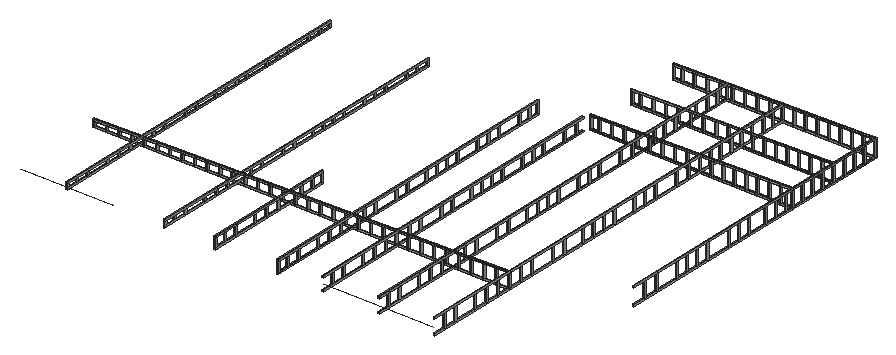
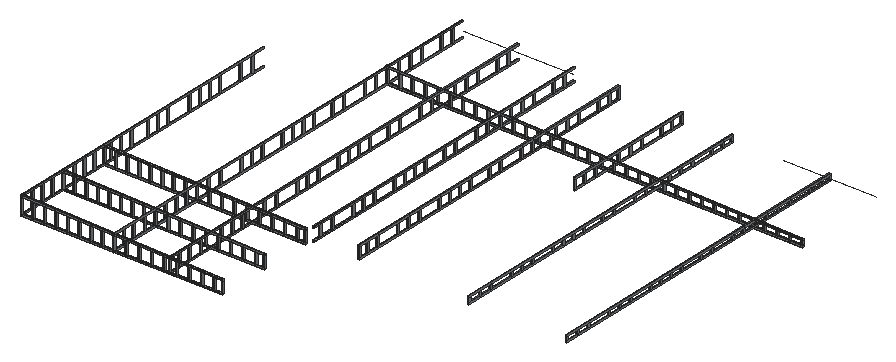
# SketchUp Ruby script. Lengths in millimetres.
U = 1.mm
M = Sketchup.active_model
def pt(a) = Geom::Point3d.new(a.map { |v| v * U })
def face(e, loops, mat)
  f = e.add_face(loops[0].map { |a| pt(a) })
  loops[1..].each { |l| e.add_face(l.map { |a| pt(a) }).erase! }
  f.material = f.back_material = mat if mat
  f
end
# faces: each face lists its corners as indices into pts; further lists are holes
def faces(e, pts, list, mat = nil) = list.each { |f| face(e, (f[0].is_a?(Array) ? f : [f]).map { |l| l.map { |i| pts[i] } }, mat) }
# xy, xz, yz: faces in a plane at the given z, y or x. An outline is a flat list of corners, or four numbers for a rectangle; further outlines are holes
def ring(l) = l.size == 4 ? [[l[0], l[1]], [l[2], l[1]], [l[2], l[3]], [l[0], l[3]]] : l.each_slice(2).to_a
def flat(e, list, mat, &to3) = list.each { |f| face(e, (f[0].is_a?(Array) ? f : [f]).map { |l| ring(l).map { |u, v| to3.(u, v) } }, mat) }
def xy(e, z, list, mat = nil) = flat(e, list, mat) { |x, y| [x, y, z] }
def xz(e, y, list, mat = nil) = flat(e, list, mat) { |x, z| [x, y, z] }
def yz(e, x, list, mat = nil) = flat(e, list, mat) { |y, z| [x, y, z] }
def lines(e, pts, list) = list.each { |a, b| e.add_line(pt(pts[a]), pt(pts[b])) }
# prism: a flat outline (further loops are holes) pulled along v
def prism(e, loops, v, mat = nil)
  f = face(e, loops, mat); d = Geom::Vector3d.new(v.map { |x| x * U })
  f.pushpull(f.normal.samedirection?(d) ? d.length : -d.length)
end
def box(e, o, s, mat = nil) = prism(e, [[o, [o[0] + s[0], o[1], o[2]], [o[0] + s[0], o[1] + s[1], o[2]], [o[0], o[1] + s[1], o[2]]]], [0, 0, s[2]], mat)
def at(x, y, z, deg = 0) = Geom::Transformation.translation(pt([x, y, z])) * Geom::Transformation.rotation(ORIGIN, Z_AXIS, deg.degrees)
def axes(o, x, y, z) = Geom::Transformation.new([*x, 0, *y, 0, *z, 0, *pt(o).to_a, 1])
def part(name) = M.definitions.add(name)
# library, detail: a bought-in or finely detailed component or shape, given as its bounding box
def library(name, o, s) = part(name).tap { |d| box(d.entities, o, s) }
def detail(e, o, s) = box(e.add_group.entities, o, s)
def put(e, d, t, mat = nil) = e.add_instance(d, t).tap { |i| i.material = mat if mat }
def group(e, t, mat = nil) = e.add_group.tap { |g| g.transformation = t; g.material = mat if mat }.entities
root = M.entities
M.materials.add("[Metal Rough]").color = [153, 157, 160]
c1 = part("Group\#8")
prism(c1.entities,[[[24013.3,85,80],[24013.3,85,831.9],[23933.3,85,830.1],[23933.3,85,80]]],[0,80,0],"[Metal Rough]")
prism(c1.entities,[[[20160.7,165,80],[20080.7,165,80],[20080.7,165,744.8],[20135.2,165,746],[20160.7,165,746.6]]],[0,-80,0],"[Metal Rough]")
prism(c1.entities,[[[20830,165,80],[20750,165,80],[20750,165,759.6],[20804.6,165,760.8],[20830,165,761.4]]],[0,-80,0],"[Metal Rough]")
prism(c1.entities,[[[18152.6,165,80],[18072.6,165,80],[18072.6,165,700.3],[18127.1,165,701.5],[18152.6,165,702.1]]],[0,-80,0],"[Metal Rough]")
prism(c1.entities,[[[21499.4,165,80],[21419.4,165,80],[21419.4,165,774.4],[21473.9,165,775.6],[21499.4,165,776.2]]],[0,-80,0],"[Metal Rough]")
prism(c1.entities,[[[19491.3,165,80],[19411.3,165,80],[19411.3,165,730],[19465.8,165,731.2],[19491.3,165,731.7]]],[0,-80,0],"[Metal Rough]")
prism(c1.entities,[[[16813.9,165,80],[16733.9,165,80],[16733.9,165,670.7],[16788.4,165,671.9],[16813.9,165,672.4]]],[0,-80,0],"[Metal Rough]")
prism(c1.entities,[[[16373.7,165,80],[16293.7,165,80],[16293.7,165,655.8],[16293.6,165,660.9],[16348.1,165,662.1],[16373.6,165,662.7],[16373.7,165,657.6]]],[0,-80,0],"[Metal Rough]")
prism(c1.entities,[[[17483.3,165,80],[17403.3,165,80],[17403.3,165,685.5],[17457.8,165,686.7],[17483.3,165,687.3]]],[0,-80,0],"[Metal Rough]")
prism(c1.entities,[[[18822,165,80],[18742,165,80],[18742,165,715.1],[18796.5,165,716.3],[18822,165,716.9]]],[0,-80,0],"[Metal Rough]")
prism(c1.entities,[[[27087.5,85,80],[27087.5,85,900],[27007.5,85,897.8],[27007.5,85,80]]],[0,80,0],"[Metal Rough]")
prism(c1.entities,[[[26472.7,165,80],[26392.7,165,80],[26392.7,165,884.6],[26472.7,165,886.4]]],[0,-80,0],"[Metal Rough]")
prism(c1.entities,[[[25857.8,165,80],[25777.8,165,80],[25777.8,165,871],[25857.8,165,872.8]]],[0,-80,0],"[Metal Rough]")
prism(c1.entities,[[[22168.7,165,80],[22088.7,165,80],[22088.8,165,789.3],[22168.8,165,791]]],[0,-80,0],"[Metal Rough]")
prism(c1.entities,[[[25243,165,80],[25163,165,80],[25163,165,857.4],[25243,165,859.1]]],[0,-80,0],"[Metal Rough]")
prism(c1.entities,[[[24628.1,165,80],[24548.1,165,80],[24548.1,165,843.7],[24628.1,165,845.5]]],[0,-80,0],"[Metal Rough]")
prism(c1.entities,[[[22783.6,85,80],[22783.6,85,804.7],[22703.6,85,802.9],[22703.6,85,80]]],[0,80,0],"[Metal Rough]")
prism(c1.entities,[[[23398.4,165,80],[23318.4,165,80],[23318.4,165,816.5],[23398.4,165,818.3]]],[0,-80,0],"[Metal Rough]")
p = [[21499.4,85,776.2],[21553.9,85,777.4]]
lines(c1.entities,p,[[0,1]])
g1 = group(c1.entities,at(0,85,0),"[Metal Rough]")
g2 = group(g1,at(0,0,300))
prism(g2,[[[27087.5,80,600],[16293.7,80,360.9],[16293.7,80,440.9],[27087.5,80,680]]],[0,-80,0])
g3 = group(g1,at(27087.5,0,0),"[Metal Rough]")
xy(g3,0,[[-10793.8,0,0,80]])
xy(g3,4,[[-10793.8,4,0,76]])
xy(g3,76,[[-10793.8,4,0,76]])
xy(g3,80,[[-10793.8,0,0,80]])
xz(g3,0,[[-10793.8,0,0,80]])
xz(g3,4,[[-10793.8,4,0,76]])
xz(g3,80,[[-10793.8,0,0,80]])
yz(g3,-10793.8,[[0,0,0,80,80,80,80,76,4,76,4,4,80,4,80,0],[4,4,80,76]])
yz(g3,0,[[[0,0,80,80],[4,4,76,76]]])
c2 = part("Group\#51")
box(c2.entities,[0,0,0],[80,17322.9,80])
c3 = part("Group\#46")
box(c3.entities,[0,0,0],[80,17322.9,80])
c4 = part("Group\#57")
box(c4.entities,[0,0,0],[80,80,820])
c5 = part("Group\#52")
box(c5.entities,[0,0,0],[80,23204,80])
c6 = part("Group\#7")
prism(c6.entities,[[[0,0,4955],[0,80,4955],[80,80,4955],[80,0,4955]],[[76,76,4955],[4,76,4955],[4,4,4955],[76,4,4955]]],[0,0,22132.5])
c7 = part("Group\#29")
box(c7.entities,[0,0,0],[80,16119.2,80])
c8 = part("Group\#49")
box(c8.entities,[0,0,0],[80,17546,80])
c9 = part("Group\#48")
box(c9.entities,[0,0,0],[80,17546,80])
p = [[17973.9,2438,3368.8],[23848.8,2438,3368.8],[1836.3,2438,3190.9],[6789.8,2438,3190.9]]
lines(root,p,[[0,1],[2,3]])
put(root,c1,at(1752.5,22725.5,3000))
g4 = group(root,at(15500.9,2438,3000))
put(g4,c2,at(0,0,0),"[Metal Rough]")
put(g4,c3,at(0,0,606.2),"[Metal Rough]")
put(g4,c4,axes([0,1326.8,80],[1,0,0],[0,1,0],[0,0,0.64174]),"[Metal Rough]")
put(g4,c4,axes([0,619.8,80],[1,0,0],[0,1,0],[0,0,0.64174]),"[Metal Rough]")
put(g4,c4,axes([0,2630.8,80],[1,0,0],[0,1,0],[0,0,0.64174]),"[Metal Rough]")
put(g4,c4,axes([0,3409.8,80],[1,0,0],[0,1,0],[0,0,0.64174]),"[Metal Rough]")
put(g4,c4,axes([0,4163.8,80],[1,0,0],[0,1,0],[0,0,0.64174]),"[Metal Rough]")
put(g4,c4,axes([0,5701.8,80],[1,0,0],[0,1,0],[0,0,0.64174]),"[Metal Rough]")
put(g4,c4,axes([0,6439.8,80],[1,0,0],[0,1,0],[0,0,0.64174]),"[Metal Rough]")
put(g4,c4,axes([0,8583.8,80],[1,0,0],[0,1,0],[0,0,0.64174]),"[Metal Rough]")
put(g4,c4,axes([0,7834.8,80],[1,0,0],[0,1,0],[0,0,0.64174]),"[Metal Rough]")
put(g4,c4,axes([0,9830.8,80],[1,0,0],[0,1,0],[0,0,0.64174]),"[Metal Rough]")
put(g4,c4,axes([0,10547.8,80],[1,0,0],[0,1,0],[0,0,0.64174]),"[Metal Rough]")
put(g4,c4,axes([0,11219.8,80],[1,0,0],[0,1,0],[0,0,0.64174]),"[Metal Rough]")
put(g4,c4,axes([0,11903.8,80],[1,0,0],[0,1,0],[0,0,0.64174]),"[Metal Rough]")
put(g4,c4,axes([0,13240.8,80],[1,0,0],[0,1,0],[0,0,0.64174]),"[Metal Rough]")
put(g4,c4,axes([0,13957.8,80],[1,0,0],[0,1,0],[0,0,0.64174]),"[Metal Rough]")
put(g4,c4,axes([0,14664.8,80],[1,0,0],[0,1,0],[0,0,0.64174]),"[Metal Rough]")
put(g4,c4,axes([0,16044.8,80],[1,0,0],[0,1,0],[0,0,0.64174]),"[Metal Rough]")
put(g4,c4,axes([0,16680.8,80],[1,0,0],[0,1,0],[0,0,0.64174]),"[Metal Rough]")
put(g4,c4,axes([0,0,80],[1,0,0],[0,1,0],[0,0,0.64174]),"[Metal Rough]")
put(g4,c4,axes([0,17242.9,80],[1,0,0],[0,1,0],[0,0,0.64174]),"[Metal Rough]")
put(root,c1,at(1756.3,19974,3000))
put(root,c1,at(1756.3,25477,3000))
g5 = group(root,at(17893.9,2438,3000))
put(g5,c2,at(0,0,0),"[Metal Rough]")
put(g5,c3,at(0,0,659.2),"[Metal Rough]")
put(g5,c4,axes([0,1326.8,80],[1,0,0],[0,1,0],[0,0,0.70638]),"[Metal Rough]")
put(g5,c4,axes([0,619.8,80],[1,0,0],[0,1,0],[0,0,0.70638]),"[Metal Rough]")
put(g5,c4,axes([0,2630.8,80],[1,0,0],[0,1,0],[0,0,0.70638]),"[Metal Rough]")
put(g5,c4,axes([0,3409.8,80],[1,0,0],[0,1,0],[0,0,0.70638]),"[Metal Rough]")
put(g5,c4,axes([0,4163.8,80],[1,0,0],[0,1,0],[0,0,0.70638]),"[Metal Rough]")
put(g5,c4,axes([0,5701.8,80],[1,0,0],[0,1,0],[0,0,0.70638]),"[Metal Rough]")
put(g5,c4,axes([0,6439.8,80],[1,0,0],[0,1,0],[0,0,0.70638]),"[Metal Rough]")
put(g5,c4,axes([0,8583.8,80],[1,0,0],[0,1,0],[0,0,0.70638]),"[Metal Rough]")
put(g5,c4,axes([0,7834.8,80],[1,0,0],[0,1,0],[0,0,0.70638]),"[Metal Rough]")
put(g5,c4,axes([0,9830.8,80],[1,0,0],[0,1,0],[0,0,0.70638]),"[Metal Rough]")
put(g5,c4,axes([0,10547.8,80],[1,0,0],[0,1,0],[0,0,0.70638]),"[Metal Rough]")
put(g5,c4,axes([0,11219.8,80],[1,0,0],[0,1,0],[0,0,0.70638]),"[Metal Rough]")
put(g5,c4,axes([0,11903.8,80],[1,0,0],[0,1,0],[0,0,0.70638]),"[Metal Rough]")
put(g5,c4,axes([0,13240.8,80],[1,0,0],[0,1,0],[0,0,0.70638]),"[Metal Rough]")
put(g5,c4,axes([0,13957.8,80],[1,0,0],[0,1,0],[0,0,0.70638]),"[Metal Rough]")
put(g5,c4,axes([0,14664.8,80],[1,0,0],[0,1,0],[0,0,0.70638]),"[Metal Rough]")
put(g5,c4,axes([0,16044.8,80],[1,0,0],[0,1,0],[0,0,0.70638]),"[Metal Rough]")
put(g5,c4,axes([0,16860.8,80],[1,0,0],[0,1,0],[0,0,0.70638]),"[Metal Rough]")
g6 = group(root,at(20871.3,2438,3000))
put(g6,c5,at(0,0,0),"[Metal Rough]")
put(g6,c5,at(0,0,725.2),"[Metal Rough]")
put(g6,c4,axes([0,1326.8,80],[1,0,0],[0,1,0],[0,0,0.78681]),"[Metal Rough]")
put(g6,c4,axes([0,619.8,80],[1,0,0],[0,1,0],[0,0,0.78681]),"[Metal Rough]")
put(g6,c4,axes([0,2630.8,80],[1,0,0],[0,1,0],[0,0,0.78681]),"[Metal Rough]")
put(g6,c4,axes([0,3409.8,80],[1,0,0],[0,1,0],[0,0,0.78681]),"[Metal Rough]")
put(g6,c4,axes([0,4163.8,80],[1,0,0],[0,1,0],[0,0,0.78681]),"[Metal Rough]")
put(g6,c4,axes([0,5701.8,80],[1,0,0],[0,1,0],[0,0,0.78681]),"[Metal Rough]")
put(g6,c4,axes([0,6439.8,80],[1,0,0],[0,1,0],[0,0,0.78681]),"[Metal Rough]")
put(g6,c4,axes([0,8583.8,80],[1,0,0],[0,1,0],[0,0,0.78681]),"[Metal Rough]")
put(g6,c4,axes([0,7834.8,80],[1,0,0],[0,1,0],[0,0,0.78681]),"[Metal Rough]")
put(g6,c4,axes([0,9830.8,80],[1,0,0],[0,1,0],[0,0,0.78681]),"[Metal Rough]")
put(g6,c4,axes([0,10547.8,80],[1,0,0],[0,1,0],[0,0,0.78681]),"[Metal Rough]")
put(g6,c4,axes([0,11219.8,80],[1,0,0],[0,1,0],[0,0,0.78681]),"[Metal Rough]")
put(g6,c4,axes([0,11903.8,80],[1,0,0],[0,1,0],[0,0,0.78681]),"[Metal Rough]")
put(g6,c4,axes([0,13240.8,80],[1,0,0],[0,1,0],[0,0,0.78681]),"[Metal Rough]")
put(g6,c4,axes([0,13957.8,80],[1,0,0],[0,1,0],[0,0,0.78681]),"[Metal Rough]")
put(g6,c4,axes([0,14664.8,80],[1,0,0],[0,1,0],[0,0,0.78681]),"[Metal Rough]")
put(g6,c4,axes([0,16044.8,80],[1,0,0],[0,1,0],[0,0,0.78681]),"[Metal Rough]")
put(g6,c4,axes([0,16860.8,80],[1,0,0],[0,1,0],[0,0,0.78681]),"[Metal Rough]")
put(g6,c4,axes([0,18313.8,80],[1,0,0],[0,1,0],[0,0,0.78681]),"[Metal Rough]")
put(g6,c4,axes([0,19693.8,80],[1,0,0],[0,1,0],[0,0,0.78681]),"[Metal Rough]")
put(g6,c4,axes([0,18980.8,80],[1,0,0],[0,1,0],[0,0,0.78681]),"[Metal Rough]")
put(g6,c4,axes([0,21064.8,80],[1,0,0],[0,1,0],[0,0,0.78681]),"[Metal Rough]")
put(g6,c4,axes([0,21831.8,80],[1,0,0],[0,1,0],[0,0,0.78681]),"[Metal Rough]")
put(g6,c4,axes([0,22478.8,80],[1,0,0],[0,1,0],[0,0,0.78681]),"[Metal Rough]")
put(g6,c4,axes([0,23124,80],[1,0,0],[0,1,0],[0,0,0.78681]),"[Metal Rough]")
g7 = group(root,at(23848.8,2438,3000))
put(g7,c5,at(0,0,0),"[Metal Rough]")
put(g7,c5,at(0,0,789.4),"[Metal Rough]")
put(g7,c4,axes([0,1326.8,80],[1,0,0],[0,1,0],[0,0,0.86507]),"[Metal Rough]")
put(g7,c4,axes([0,619.8,80],[1,0,0],[0,1,0],[0,0,0.86507]),"[Metal Rough]")
put(g7,c4,axes([0,2630.8,80],[1,0,0],[0,1,0],[0,0,0.86507]),"[Metal Rough]")
put(g7,c4,axes([0,3409.8,80],[1,0,0],[0,1,0],[0,0,0.86507]),"[Metal Rough]")
put(g7,c4,axes([0,4163.8,80],[1,0,0],[0,1,0],[0,0,0.86507]),"[Metal Rough]")
put(g7,c4,axes([0,5701.8,80],[1,0,0],[0,1,0],[0,0,0.86507]),"[Metal Rough]")
put(g7,c4,axes([0,6439.8,80],[1,0,0],[0,1,0],[0,0,0.86507]),"[Metal Rough]")
put(g7,c4,axes([0,8583.8,80],[1,0,0],[0,1,0],[0,0,0.86507]),"[Metal Rough]")
put(g7,c4,axes([0,7834.8,80],[1,0,0],[0,1,0],[0,0,0.86507]),"[Metal Rough]")
put(g7,c4,axes([0,9830.8,80],[1,0,0],[0,1,0],[0,0,0.86507]),"[Metal Rough]")
put(g7,c4,axes([0,10547.8,80],[1,0,0],[0,1,0],[0,0,0.86507]),"[Metal Rough]")
put(g7,c4,axes([0,11219.8,80],[1,0,0],[0,1,0],[0,0,0.86507]),"[Metal Rough]")
put(g7,c4,axes([0,11903.8,80],[1,0,0],[0,1,0],[0,0,0.86507]),"[Metal Rough]")
put(g7,c4,axes([0,13240.8,80],[1,0,0],[0,1,0],[0,0,0.86507]),"[Metal Rough]")
put(g7,c4,axes([0,13957.8,80],[1,0,0],[0,1,0],[0,0,0.86507]),"[Metal Rough]")
put(g7,c4,axes([0,14664.8,80],[1,0,0],[0,1,0],[0,0,0.86507]),"[Metal Rough]")
put(g7,c4,axes([0,16044.8,80],[1,0,0],[0,1,0],[0,0,0.86507]),"[Metal Rough]")
put(g7,c4,axes([0,16860.8,80],[1,0,0],[0,1,0],[0,0,0.86507]),"[Metal Rough]")
put(g7,c4,axes([0,18313.8,80],[1,0,0],[0,1,0],[0,0,0.86507]),"[Metal Rough]")
put(g7,c4,axes([0,19693.8,80],[1,0,0],[0,1,0],[0,0,0.86507]),"[Metal Rough]")
put(g7,c4,axes([0,18980.8,80],[1,0,0],[0,1,0],[0,0,0.86507]),"[Metal Rough]")
put(g7,c4,axes([0,21064.8,80],[1,0,0],[0,1,0],[0,0,0.86507]),"[Metal Rough]")
put(g7,c4,axes([0,21831.8,80],[1,0,0],[0,1,0],[0,0,0.86507]),"[Metal Rough]")
put(g7,c4,axes([0,22478.8,80],[1,0,0],[0,1,0],[0,0,0.86507]),"[Metal Rough]")
g8 = group(root,at(12150,2438,3000))
g9 = group(g8,at(0,0,0),"[Metal Rough]")
box(g9,[0,0,0],[80,7145.8,80])
g10 = group(g8,at(0,0,532),"[Metal Rough]")
box(g10,[0,0,0],[80,7145.8,80])
put(g8,c4,axes([0,1326.8,80],[1,0,0],[0,1,0],[0,0,0.55122]),"[Metal Rough]")
put(g8,c4,axes([0,619.8,80],[1,0,0],[0,1,0],[0,0,0.55122]),"[Metal Rough]")
put(g8,c4,axes([0,2630.8,80],[1,0,0],[0,1,0],[0,0,0.55122]),"[Metal Rough]")
put(g8,c4,axes([0,3409.8,80],[1,0,0],[0,1,0],[0,0,0.55122]),"[Metal Rough]")
put(g8,c4,axes([0,4163.8,80],[1,0,0],[0,1,0],[0,0,0.55122]),"[Metal Rough]")
put(g8,c4,axes([0,5701.8,80],[1,0,0],[0,1,0],[0,0,0.55122]),"[Metal Rough]")
put(g8,c4,axes([0,6439.8,80],[1,0,0],[0,1,0],[0,0,0.55122]),"[Metal Rough]")
put(g8,c4,axes([0,7084.8,80],[1,0,0],[0,1,0],[0,0,0.55122]),"[Metal Rough]")
put(g8,c4,axes([0,0,80],[1,0,0],[0,1,0],[0,0,0.55122]),"[Metal Rough]")
g11 = group(root,at(1756.3,7283,3000))
prism(g11,[[[6104.2,85,80],[6104.2,85,435.2],[6078.7,85,434.6],[6024.2,85,433.4],[6024.2,85,80]]],[0,80,0],"[Metal Rough]")
prism(g11,[[[7442.9,85,80],[7442.9,85,464.9],[7417.4,85,464.3],[7362.9,85,463.1],[7362.9,85,80]]],[0,80,0],"[Metal Rough]")
prism(g11,[[[6773.6,85,80],[6773.6,85,450],[6748.1,85,449.5],[6693.6,85,448.3],[6693.6,85,80]]],[0,80,0],"[Metal Rough]")
prism(g11,[[[8112.3,85,80],[8112.3,85,479.7],[8086.8,85,479.1],[8032.3,85,477.9],[8032.3,85,80]]],[0,80,0],"[Metal Rough]")
prism(g11,[[[5434.8,85,80],[5434.8,85,420.4],[5409.4,85,419.8],[5354.8,85,418.6],[5354.8,85,80]]],[0,80,0],"[Metal Rough]")
prism(g11,[[[4096.1,85,80],[4096.1,85,390.7],[4070.6,85,390.2],[4016.1,85,388.9],[4016.1,85,80]]],[0,80,0],"[Metal Rough]")
prism(g11,[[[1418.7,165,80],[1338.7,165,80],[1338.7,165,329.6],[1393.2,165,330.9],[1418.7,165,331.4]]],[0,-80,0],"[Metal Rough]")
prism(g11,[[[3426.8,165,80],[3346.8,165,80],[3346.8,165,374.1],[3401.3,165,375.3],[3426.8,165,375.9]]],[0,-80,0],"[Metal Rough]")
prism(g11,[[[2757.4,165,80],[2677.4,165,80],[2677.4,165,359.3],[2731.9,165,360.5],[2757.4,165,361.1]]],[0,-80,0],"[Metal Rough]")
prism(g11,[[[2088.1,165,80],[2008.1,165,80],[2008.1,165,344.5],[2062.6,165,345.7],[2088.1,165,346.2]]],[0,-80,0],"[Metal Rough]")
prism(g11,[[[4765.5,85,80],[4765.5,85,405.5],[4740,85,405],[4685.5,85,403.8],[4685.5,85,80]]],[0,80,0],"[Metal Rough]")
prism(g11,[[[80,85,80],[80,85,301.8],[0,85,300],[0,85,80]]],[0,80,0],"[Metal Rough]")
prism(g11,[[[749.4,85,80],[749.4,85,316.6],[669.4,85,314.8],[669.4,85,80]]],[0,80,0],"[Metal Rough]")
prism(g11,[[[12128.4,85,80],[12128.4,85,568.6],[12102.9,85,568.1],[12048.4,85,566.9],[12048.4,85,80]]],[0,80,0],"[Metal Rough]")
prism(g11,[[[10120.3,165,80],[10040.3,165,80],[10040.3,165,522.4],[10094.9,165,523.6],[10120.3,165,524.2]]],[0,-80,0],"[Metal Rough]")
prism(g11,[[[12797.8,85,80],[12797.8,85,583.5],[12772.3,85,582.9],[12717.8,85,581.7],[12717.8,85,80]]],[0,80,0],"[Metal Rough]")
prism(g11,[[[20160.7,165,80],[20080.7,165,80],[20080.7,165,744.8],[20135.2,165,746],[20160.7,165,746.6]]],[0,-80,0],"[Metal Rough]")
prism(g11,[[[20830,165,80],[20750,165,80],[20750,165,759.6],[20804.6,165,760.8],[20830,165,761.4]]],[0,-80,0],"[Metal Rough]")
prism(g11,[[[18152.6,165,80],[18072.6,165,80],[18072.6,165,700.3],[18127.1,165,701.5],[18152.6,165,702.1]]],[0,-80,0],"[Metal Rough]")
prism(g11,[[[21499.4,165,80],[21419.4,165,80],[21419.4,165,774.4],[21473.9,165,775.6],[21499.4,165,776.2]]],[0,-80,0],"[Metal Rough]")
prism(g11,[[[15475.2,165,80],[15395.2,165,80],[15395.2,165,641],[15449.7,165,642.2],[15475.2,165,642.8]]],[0,-80,0],"[Metal Rough]")
prism(g11,[[[19491.3,165,80],[19411.3,165,80],[19411.3,165,730],[19465.8,165,731.2],[19491.3,165,731.7]]],[0,-80,0],"[Metal Rough]")
prism(g11,[[[16813.9,165,80],[16733.9,165,80],[16733.9,165,670.7],[16788.4,165,671.9],[16813.9,165,672.4]]],[0,-80,0],"[Metal Rough]")
prism(g11,[[[16144.5,165,80],[16064.5,165,80],[16064.5,165,655.8],[16119.1,165,657],[16144.5,165,657.6]]],[0,-80,0],"[Metal Rough]")
prism(g11,[[[17483.3,165,80],[17403.3,165,80],[17403.3,165,685.5],[17457.8,165,686.7],[17483.3,165,687.3]]],[0,-80,0],"[Metal Rough]")
prism(g11,[[[14805.8,165,80],[14725.8,165,80],[14725.8,165,626.2],[14780.3,165,627.4],[14805.8,165,627.9]]],[0,-80,0],"[Metal Rough]")
prism(g11,[[[18822,165,80],[18742,165,80],[18742,165,715.1],[18796.5,165,716.3],[18822,165,716.9]]],[0,-80,0],"[Metal Rough]")
prism(g11,[[[10789.7,165,80],[10709.7,165,80],[10709.7,165,537.2],[10764.2,165,538.4],[10789.7,165,539]]],[0,-80,0],"[Metal Rough]")
prism(g11,[[[8781.6,165,80],[8701.6,165,80],[8701.6,165,492.7],[8756.1,165,493.9],[8781.6,165,494.5]]],[0,-80,0],"[Metal Rough]")
prism(g11,[[[9451,165,80],[9371,165,80],[9371,165,507.6],[9425.5,165,508.8],[9451,165,509.3]]],[0,-80,0],"[Metal Rough]")
prism(g11,[[[13467.1,165,80],[13387.1,165,80],[13387.1,165,596.5],[13441.6,165,597.7],[13467.1,165,598.3]]],[0,-80,0],"[Metal Rough]")
prism(g11,[[[14136.5,165,80],[14056.5,165,80],[14056.5,165,611.3],[14111,165,612.6],[14136.5,165,613.1]]],[0,-80,0],"[Metal Rough]")
prism(g11,[[[11459.1,165,80],[11379.1,165,80],[11379.1,165,552],[11433.6,165,553.2],[11459.1,165,553.8]]],[0,-80,0],"[Metal Rough]")
prism(g11,[[[22172.5,165,80],[22092.5,165,80],[22092.5,165,788.5],[22172.5,165,790.2]]],[0,-80,0],"[Metal Rough]")
p = [[21499.4,85,776.2],[21553.9,85,777.4]]
lines(g11,p,[[0,1]])
g12 = group(g11,at(0,85,0),"[Metal Rough]")
g13 = group(g12,at(0,0,300))
prism(g13,[[[0,80,80],[22132.5,80,570.3],[22172.5,80,570.3],[22172.5,80,490.2],[22132.5,80,490.2],[0,80,0]]],[0,-80,0])
put(g12,c6,axes([27087.5,0,0],[0,0,1],[0,1,0],[-1,0,0]),"[Metal Rough]")
g14 = group(root,at(28763.8,9522.8,3000))
g15 = group(g14,at(0,11217.2,80))
put(g15,c4,at(0,1336,0),"[Metal Rough]")
put(g15,c4,at(0,2775,0),"[Metal Rough]")
put(g15,c4,at(0,4111,0),"[Metal Rough]")
put(g15,c4,at(0,3443,0),"[Metal Rough]")
put(g15,c4,at(0,668,0),"[Metal Rough]")
put(g15,c4,at(0,0,0),"[Metal Rough]")
put(g15,c4,at(0,-1117,0),"[Metal Rough]")
put(g15,c4,at(0,-1785,0),"[Metal Rough]")
put(g15,c4,at(0,-2453,0),"[Metal Rough]")
put(g15,c4,at(0,-4232,0),"[Metal Rough]")
put(g15,c4,at(0,-3564,0),"[Metal Rough]")
put(g15,c4,at(0,-4900,0),"[Metal Rough]")
put(g15,c4,at(0,-7693,0),"[Metal Rough]")
put(g15,c4,at(0,-7025,0),"[Metal Rough]")
put(g15,c4,at(0,-6357,0),"[Metal Rough]")
put(g15,c4,at(0,-8364,0),"[Metal Rough]")
put(g15,c4,at(0,-9727,0),"[Metal Rough]")
put(g15,c4,at(0,-10515,0),"[Metal Rough]")
put(g14,c7,at(0,0,900),"[Metal Rough]")
put(g14,c7,at(0,0,0),"[Metal Rough]")
g16 = group(root,at(4273,2438,3080))
put(g16,c8,at(0,0,0),"[Metal Rough]")
put(g16,c9,at(0,0,277.5),"[Metal Rough]")
put(g16,c4,axes([0,1326.8,80],[1,0,0],[0,1,0],[0,0,0.24089]),"[Metal Rough]")
put(g16,c4,axes([0,619.8,80],[1,0,0],[0,1,0],[0,0,0.24089]),"[Metal Rough]")
put(g16,c4,axes([0,2630.8,80],[1,0,0],[0,1,0],[0,0,0.24089]),"[Metal Rough]")
put(g16,c4,axes([0,3409.8,80],[1,0,0],[0,1,0],[0,0,0.24089]),"[Metal Rough]")
put(g16,c4,axes([0,4163.8,80],[1,0,0],[0,1,0],[0,0,0.24089]),"[Metal Rough]")
put(g16,c4,axes([0,5701.8,80],[1,0,0],[0,1,0],[0,0,0.24089]),"[Metal Rough]")
put(g16,c4,axes([0,6439.8,80],[1,0,0],[0,1,0],[0,0,0.24089]),"[Metal Rough]")
put(g16,c4,axes([0,8583.8,80],[1,0,0],[0,1,0],[0,0,0.24089]),"[Metal Rough]")
put(g16,c4,axes([0,7834.8,80],[1,0,0],[0,1,0],[0,0,0.24089]),"[Metal Rough]")
put(g16,c4,axes([0,9830.8,80],[1,0,0],[0,1,0],[0,0,0.24089]),"[Metal Rough]")
put(g16,c4,axes([0,10547.8,80],[1,0,0],[0,1,0],[0,0,0.24089]),"[Metal Rough]")
put(g16,c4,axes([0,11219.8,80],[1,0,0],[0,1,0],[0,0,0.24089]),"[Metal Rough]")
put(g16,c4,axes([0,11903.8,80],[1,0,0],[0,1,0],[0,0,0.24089]),"[Metal Rough]")
put(g16,c4,axes([0,13240.8,80],[1,0,0],[0,1,0],[0,0,0.24089]),"[Metal Rough]")
put(g16,c4,axes([0,13957.8,80],[1,0,0],[0,1,0],[0,0,0.24089]),"[Metal Rough]")
put(g16,c4,axes([0,14664.8,80],[1,0,0],[0,1,0],[0,0,0.24089]),"[Metal Rough]")
put(g16,c4,axes([0,16044.8,80],[1,0,0],[0,1,0],[0,0,0.24089]),"[Metal Rough]")
put(g16,c4,axes([0,16762.8,80],[1,0,0],[0,1,0],[0,0,0.24089]),"[Metal Rough]")
put(g16,c4,axes([0,17466,80],[1,0,0],[0,1,0],[0,0,0.24089]),"[Metal Rough]")
put(g16,c4,axes([0,0,80],[1,0,0],[0,1,0],[0,0,0.24089]),"[Metal Rough]")
g17 = group(root,at(9469.9,2438,3080))
put(g17,c8,at(0,0,0),"[Metal Rough]")
put(g17,c9,at(0,0,312.6),"[Metal Rough]")
put(g17,c4,axes([0,1326.8,80],[1,0,0],[0,1,0],[0,0,0.28368]),"[Metal Rough]")
put(g17,c4,axes([0,619.8,80],[1,0,0],[0,1,0],[0,0,0.28368]),"[Metal Rough]")
put(g17,c4,axes([0,2630.8,80],[1,0,0],[0,1,0],[0,0,0.28368]),"[Metal Rough]")
put(g17,c4,axes([0,3409.8,80],[1,0,0],[0,1,0],[0,0,0.28368]),"[Metal Rough]")
put(g17,c4,axes([0,4163.8,80],[1,0,0],[0,1,0],[0,0,0.28368]),"[Metal Rough]")
put(g17,c4,axes([0,5701.8,80],[1,0,0],[0,1,0],[0,0,0.28368]),"[Metal Rough]")
put(g17,c4,axes([0,6439.8,80],[1,0,0],[0,1,0],[0,0,0.28368]),"[Metal Rough]")
put(g17,c4,axes([0,8583.8,80],[1,0,0],[0,1,0],[0,0,0.28368]),"[Metal Rough]")
put(g17,c4,axes([0,7834.8,80],[1,0,0],[0,1,0],[0,0,0.28368]),"[Metal Rough]")
put(g17,c4,axes([0,9830.8,80],[1,0,0],[0,1,0],[0,0,0.28368]),"[Metal Rough]")
put(g17,c4,axes([0,10547.8,80],[1,0,0],[0,1,0],[0,0,0.28368]),"[Metal Rough]")
put(g17,c4,axes([0,11219.8,80],[1,0,0],[0,1,0],[0,0,0.28368]),"[Metal Rough]")
put(g17,c4,axes([0,11903.8,80],[1,0,0],[0,1,0],[0,0,0.28368]),"[Metal Rough]")
put(g17,c4,axes([0,13240.8,80],[1,0,0],[0,1,0],[0,0,0.28368]),"[Metal Rough]")
put(g17,c4,axes([0,13957.8,80],[1,0,0],[0,1,0],[0,0,0.28368]),"[Metal Rough]")
put(g17,c4,axes([0,14664.8,80],[1,0,0],[0,1,0],[0,0,0.28368]),"[Metal Rough]")
put(g17,c4,axes([0,16044.8,80],[1,0,0],[0,1,0],[0,0,0.28368]),"[Metal Rough]")
put(g17,c4,axes([0,16762.8,80],[1,0,0],[0,1,0],[0,0,0.28368]),"[Metal Rough]")
put(g17,c4,axes([0,17466,80],[1,0,0],[0,1,0],[0,0,0.28368]),"[Metal Rough]")
put(g17,c4,axes([0,0,80],[1,0,0],[0,1,0],[0,0,0.28368]),"[Metal Rough]")
